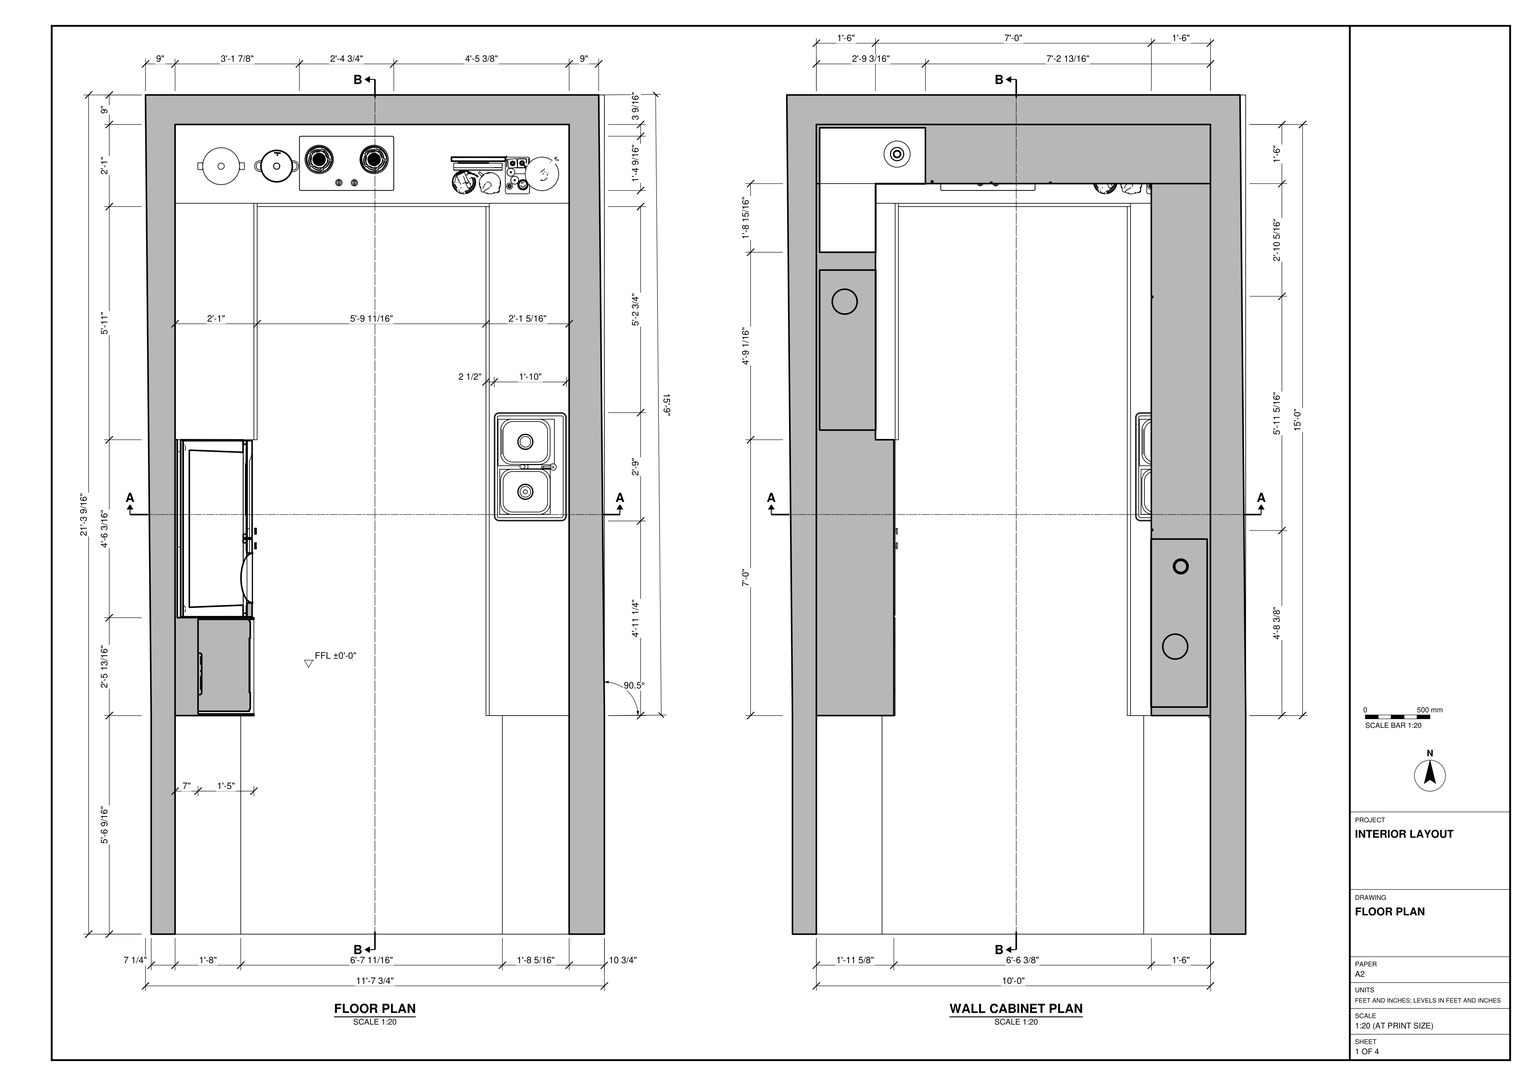
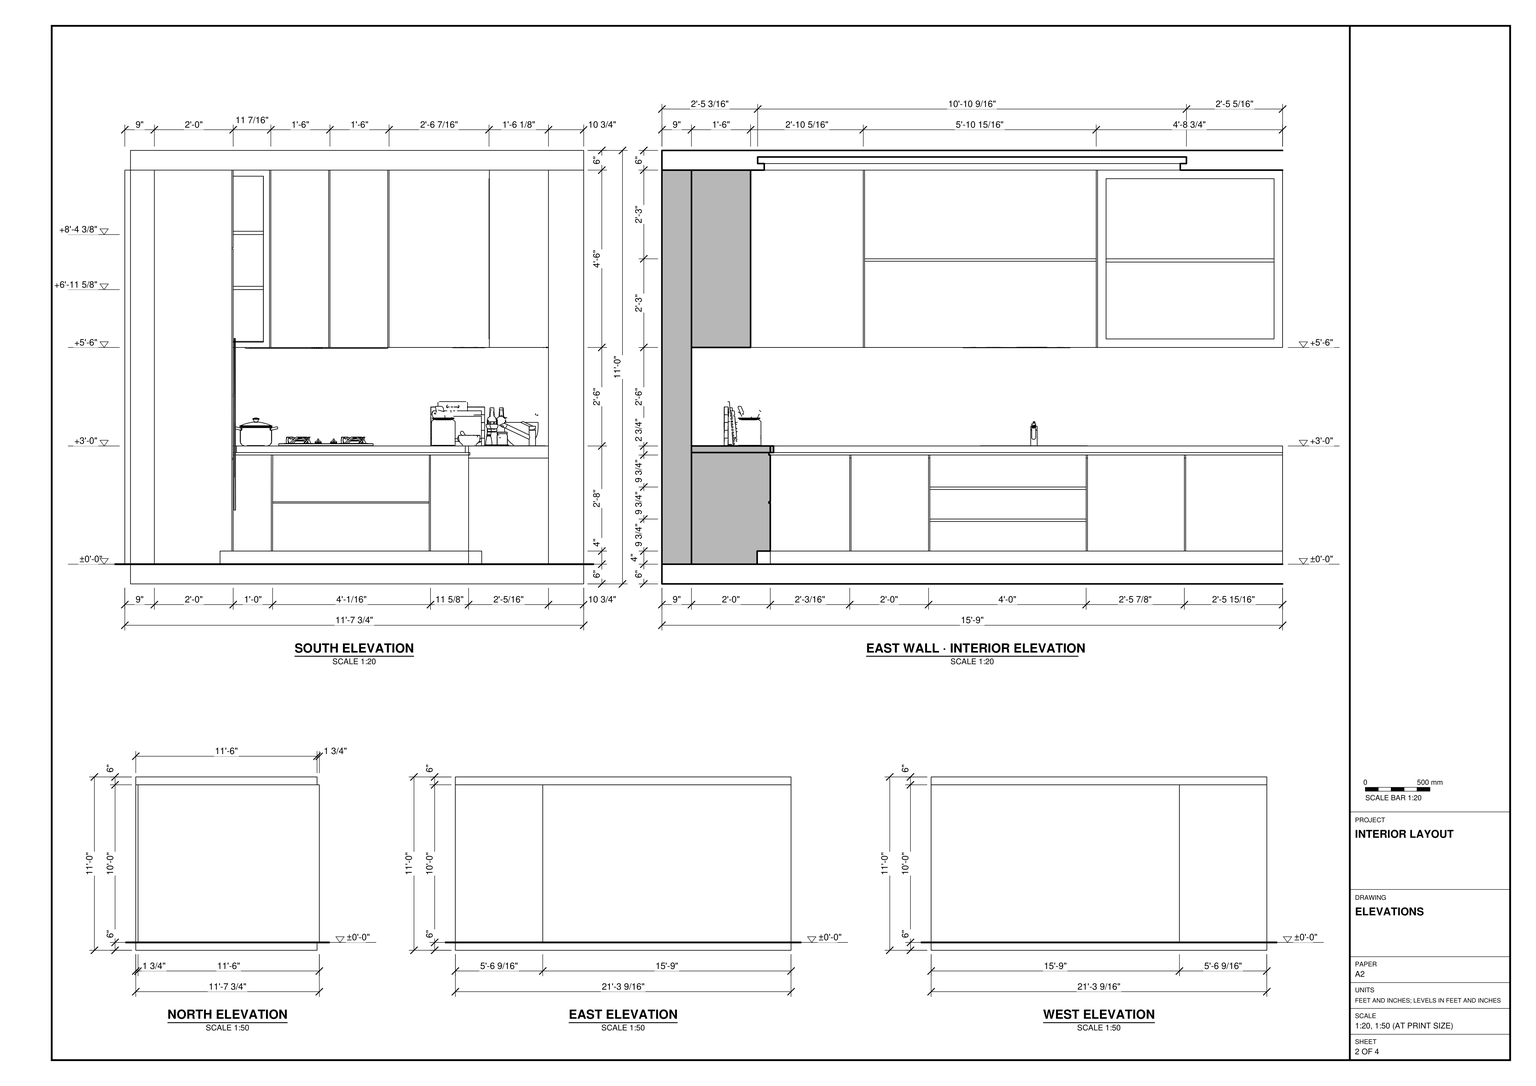
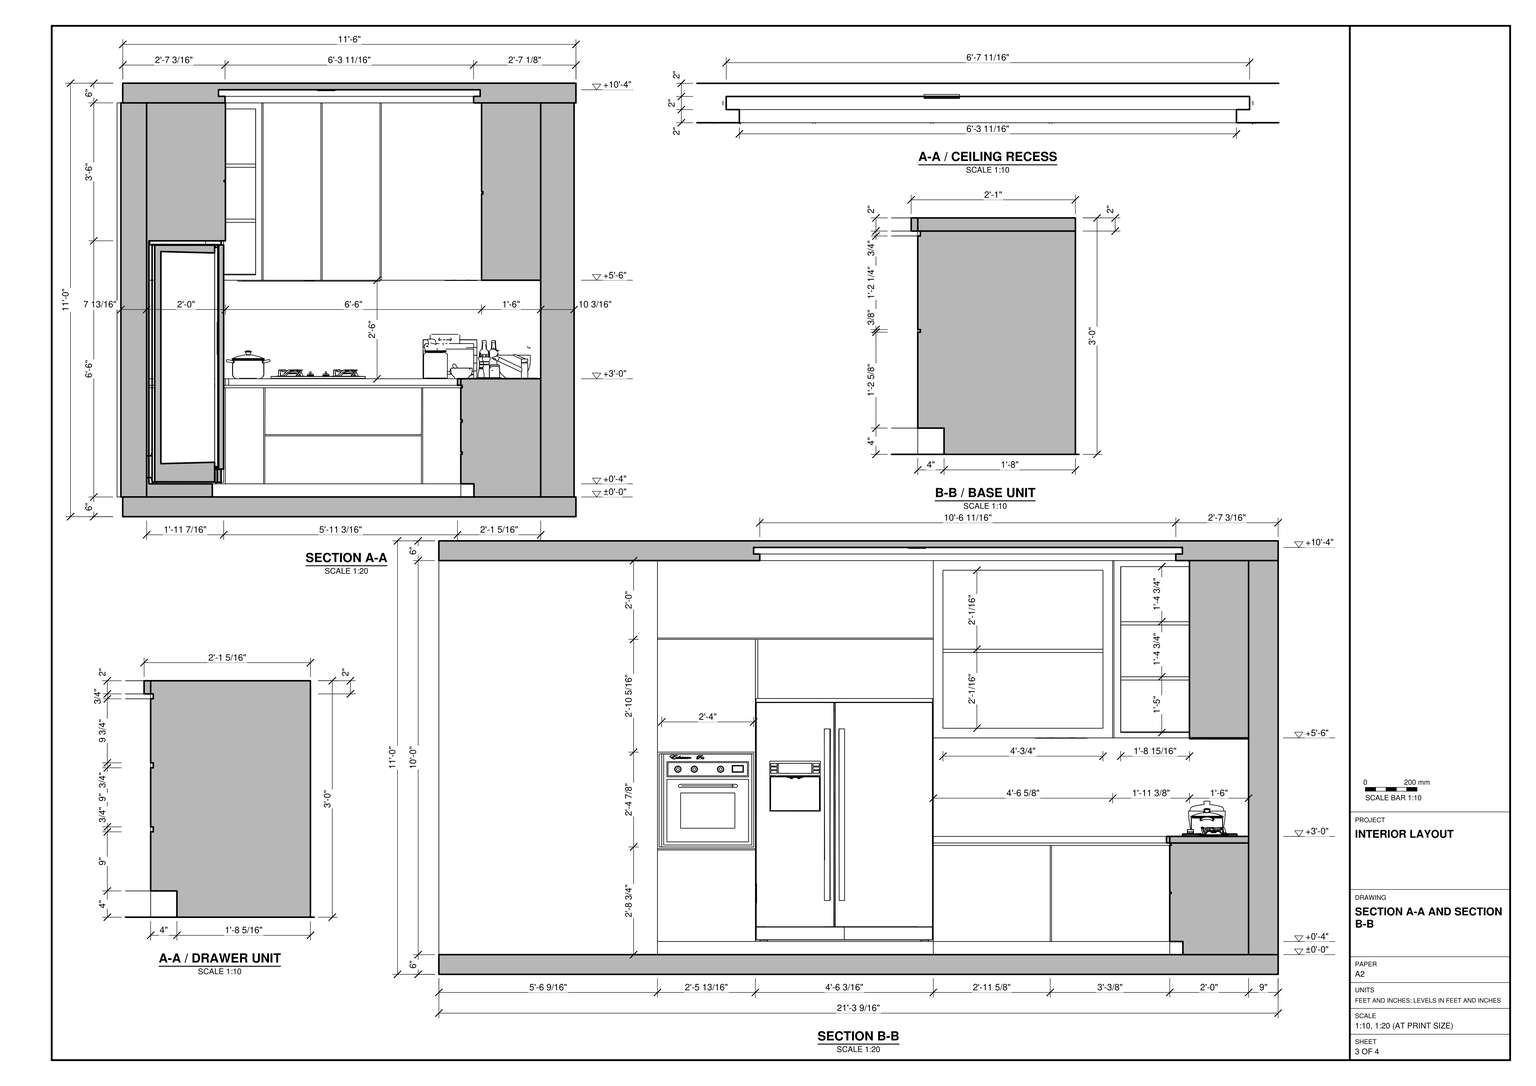
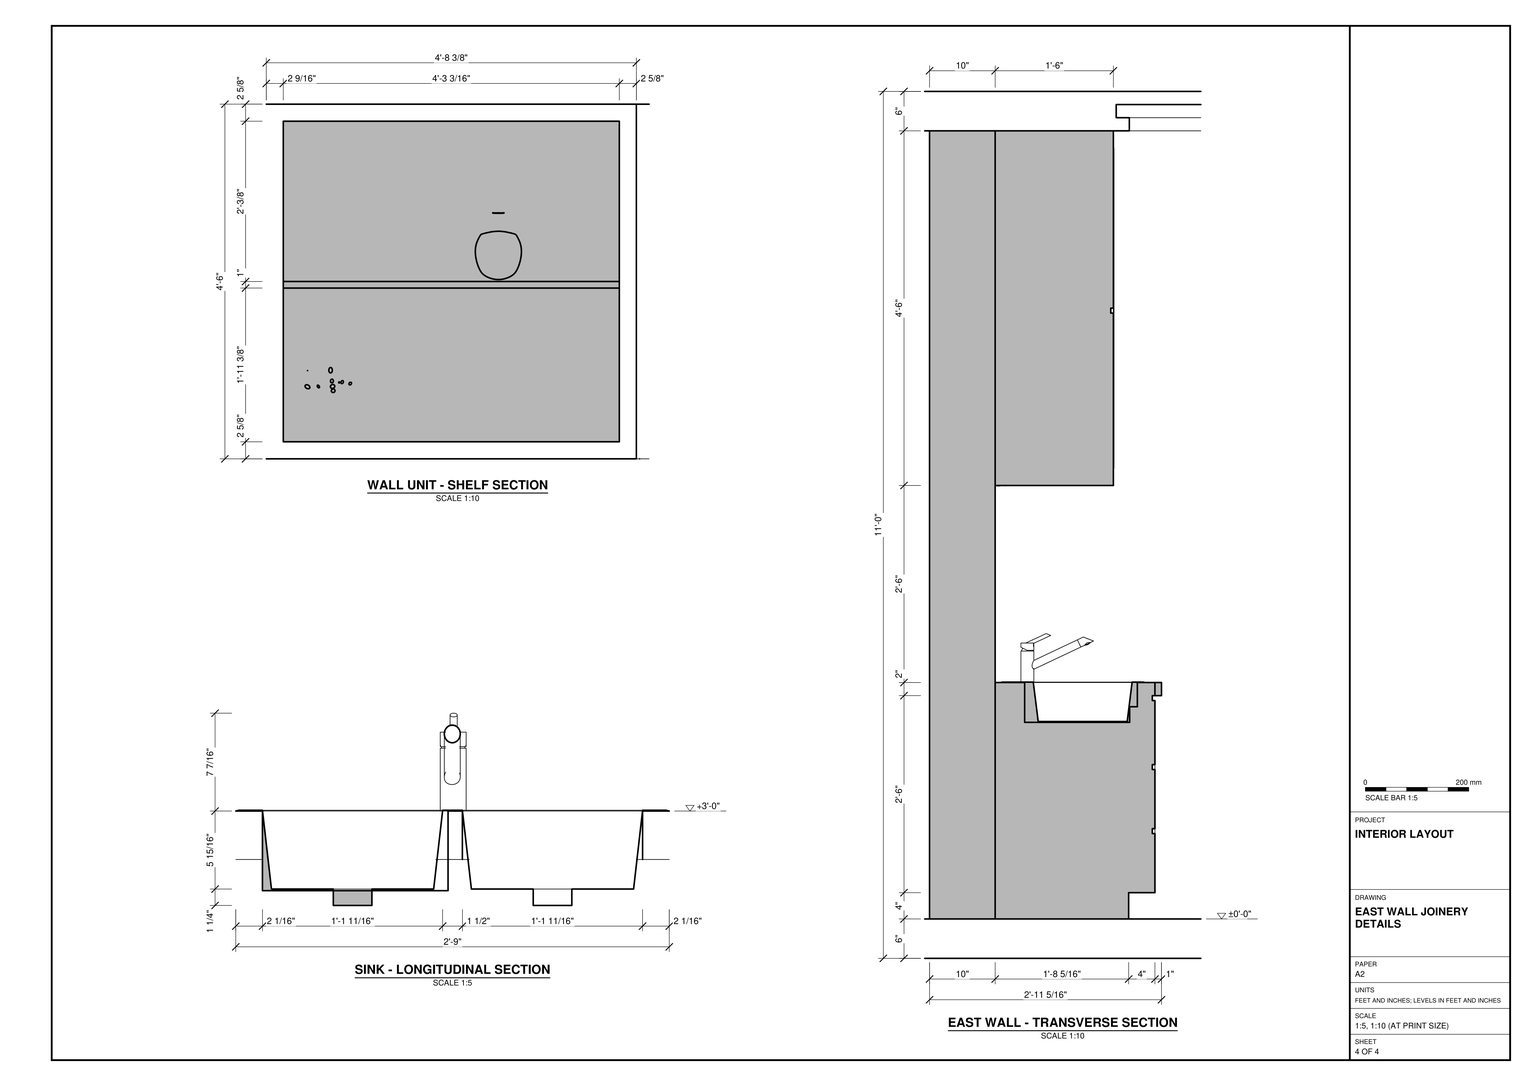
Build the kitchen interior in SketchUp using task_files/diagram_01.pdf. Work in feet and inches. The overall model is 11'-7 3/4" wide, 21'-3 9/16" long and 11'-0" high, with a single finished floor level at ±0'-0".

Model the floor slab, rear wall, side walls and ceiling slab. Follow the wall thicknesses and slight changes in alignment shown on the floor plan, leaving the front end open. Use the sections to form the stepped recess in the underside of the ceiling.

Fit the kitchen along the rear wall and both side walls, leaving the central aisle and the approach from the open end clear. Set the worktops at +3'-0". Place the cooktop on the rear run, the sink and tap on the right, and the tall oven and refrigerator bays on the left. Use the floor plan for the base units and the separate wall cabinet plan for the overhead units. Follow the elevations and sections for the drawer divisions, recessed plinths, cabinet fronts and open shelves. Appliances, cookware and other loose items may be any suitable library components.

Keep the walls, slabs and each joinery or furniture piece in separate groups or components, and use components for repeated parts. Save one SketchUp model as output_files/u_shaped_kitchen_with_cabinets_and_recessed_ceiling.skp.

# SketchUp Ruby script. Lengths in inches.
U = 1.inch
M = Sketchup.active_model
def pt(a) = Geom::Point3d.new(a.map { |v| v * U })
def face(e, loops, mat)
  f = e.add_face(loops[0].map { |a| pt(a) })
  loops[1..].each { |l| e.add_face(l.map { |a| pt(a) }).erase! }
  f.material = f.back_material = mat if mat
  f
end
# faces: each face lists its corners as indices into pts; further lists are holes
def faces(e, pts, list, mat = nil) = list.each { |f| face(e, (f[0].is_a?(Array) ? f : [f]).map { |l| l.map { |i| pts[i] } }, mat) }
# xy, xz, yz: faces in a plane at the given z, y or x. An outline is a flat list of corners, or four numbers for a rectangle; further outlines are holes
def ring(l) = l.size == 4 ? [[l[0], l[1]], [l[2], l[1]], [l[2], l[3]], [l[0], l[3]]] : l.each_slice(2).to_a
def flat(e, list, mat, &to3) = list.each { |f| face(e, (f[0].is_a?(Array) ? f : [f]).map { |l| ring(l).map { |u, v| to3.(u, v) } }, mat) }
def xy(e, z, list, mat = nil) = flat(e, list, mat) { |x, y| [x, y, z] }
def xz(e, y, list, mat = nil) = flat(e, list, mat) { |x, z| [x, y, z] }
def yz(e, x, list, mat = nil) = flat(e, list, mat) { |y, z| [x, y, z] }
def lines(e, pts, list) = list.each { |a, b| e.add_line(pt(pts[a]), pt(pts[b])) }
# prism: a flat outline (further loops are holes) pulled along v
def prism(e, loops, v, mat = nil)
  f = face(e, loops, mat); d = Geom::Vector3d.new(v.map { |x| x * U })
  f.pushpull(f.normal.samedirection?(d) ? d.length : -d.length)
end
def box(e, o, s, mat = nil) = prism(e, [[o, [o[0] + s[0], o[1], o[2]], [o[0] + s[0], o[1] + s[1], o[2]], [o[0], o[1] + s[1], o[2]]]], [0, 0, s[2]], mat)
def at(x, y, z, deg = 0) = Geom::Transformation.translation(pt([x, y, z])) * Geom::Transformation.rotation(ORIGIN, Z_AXIS, deg.degrees)
def axes(o, x, y, z) = Geom::Transformation.new([*x, 0, *y, 0, *z, 0, *pt(o).to_a, 1])
def part(name) = M.definitions.add(name)
# library, detail: a bought-in or finely detailed component or shape, given as its bounding box
def library(name, o, s) = part(name).tap { |d| box(d.entities, o, s) }
def detail(e, o, s) = box(e.add_group.entities, o, s)
def put(e, d, t, mat = nil) = e.add_instance(d, t).tap { |i| i.material = mat if mat }
def group(e, t, mat = nil) = e.add_group.tap { |g| g.transformation = t; g.material = mat if mat }.entities
root = M.entities
M.materials.add("Emissive").color = [239, 233, 180]
M.materials.add("Generic\#1").color = [204, 216, 199]
M.materials.add("Generic\#2").color = [83, 96, 74]
M.materials.add("Tiles Simple 02 100cm").color = [183, 183, 183]
M.materials.add("W147Z490B75_NILAYA MODERNISTA 32219 ROLL B75").color = [233, 234, 228]
M.materials.add("Whitewood Highgloss 300cm").color = [205, 205, 205]
M.materials.add("[Translucent Glass Gray]").color = [128, 128, 128]
M.materials["[Translucent Glass Gray]"].alpha = 0.5
M.materials.add("[Wood Veneer 02]").color = [186, 125, 89]
M.materials.add("[Wood Veneer 02]1").color = [188, 127, 90]
c1 = library("Untitled",[27.97,43.14,0],[33,22,16.3])
c2 = library("Rangemaaster flat hood",[-3.82,0.71,0],[43.23,19.01,40.35])
c3 = library("Lidded cooking pot",[0,0,0],[14.16,11.29,10.74])
c4 = part("Tlon Cubo 860 Ceiling 152 005")
xy(c4.entities,-3.04,[[-16.54,-16.54,-16.54,16.54,16.54,-16.54],[16.54,-16.54,-16.54,16.54,16.54,16.54]])
xy(c4.entities,0,[[-16.93,-16.93,16.93,-16.93,-16.93,16.93],[16.93,-16.93,16.93,16.93,-16.93,16.93]])
xz(c4.entities,-16.93,[[-16.93,-3.79,16.93,-3.79,-16.93,0],[16.93,-3.79,16.93,0,-16.93,0]])
xz(c4.entities,-16.3,[[-16.3,-3.66,-16.3,-3.24,16.3,-3.24],[-16.3,-3.66,16.3,-3.24,16.3,-3.66]])
xz(c4.entities,16.3,[[-16.3,-3.66,16.3,-3.24,-16.3,-3.24],[-16.3,-3.66,16.3,-3.66,16.3,-3.24]])
xz(c4.entities,16.93,[[-16.93,-3.79,-16.93,0,16.93,0],[-16.93,-3.79,16.93,0,16.93,-3.79]])
yz(c4.entities,-16.93,[[-16.93,-3.79,-16.93,0,16.93,0],[-16.93,-3.79,16.93,0,16.93,-3.79]])
yz(c4.entities,-16.3,[[-16.3,-3.66,16.3,-3.66,-16.3,-3.24],[16.3,-3.66,16.3,-3.24,-16.3,-3.24]])
yz(c4.entities,16.3,[[-16.3,-3.66,-16.3,-3.24,16.3,-3.66],[16.3,-3.66,-16.3,-3.24,16.3,-3.24]])
yz(c4.entities,16.93,[[-16.93,-3.79,16.93,-3.79,-16.93,0],[16.93,-3.79,16.93,0,-16.93,0]])
p = [[-16.93,-16.93,-3.79],[-16.93,16.93,-3.79],[-16.3,16.3,-3.66],[-16.3,-16.3,-3.66],[16.93,-16.93,-3.79],[16.3,-16.3,-3.66],
  [16.93,16.93,-3.79],[16.3,16.3,-3.66]]
faces(c4.entities,p,[[0,1,2],[2,3,0],[4,0,3],[3,5,4],[6,4,5],[5,7,6],[2,1,6],[6,7,2]])
c5 = library("Refrigerator 10-13",[-17.84,-12.49,0],[35.68,25.01,72.43])
c6 = library("kitchen utensils",[0,0,0],[25.84,8.08,11.16])
c7 = library("GasStove_Black",[0,0,0],[28.74,16.54,2.72])
c8 = library("现代小盆栽植物盆景多肉植物\#1",[493.55,-214.42,68.59],[116.32,134.38,44.63])
c9 = library("Kitchen oven",[-66.9,9.58,0],[22.04,24,22.83])
c10 = library("kitchen+utensil",[-39.88,-27.4,0],[79.77,28.4,32.96])
c11 = library("Kitchen Utensils - Pot",[14.77,-5.37,0.11],[13.29,9.84,8.54])
c12 = library("Gagri",[-4.64,1.37,-0.81],[22.18,22.19,29.95])
c13 = library("Group\#3",[-0.5,-0.5,0],[80.6875,131.5625,2])
c14 = part("Group\#34")
xy(c14.entities,0,[[0,0,0.1,48.73]])
xy(c14.entities,48.13,[[0,0,0.1,48.73]])
xz(c14.entities,0,[[0,0,0.1,9.0625],[0,9.0625,0.1,48.13]])
xz(c14.entities,48.73,[[0,0,0.1,48.13]])
yz(c14.entities,0,[[0,0,48.73,48.13]],"[Translucent Glass Gray]")
yz(c14.entities,0.1,[[0,0,48.73,48.13]],"[Translucent Glass Gray]")
c15 = library("Group\#35",[-0.5,-0.5,-0.1],[2,79,0.2])
c16 = library("Group\#36",[-0.5,-0.5,-0.1],[2,18,0.2])
c17 = library("Group\#82",[-0.5,-0.5,-0.1],[28.04,2,0.2])
c18 = library("Group\#83",[-0.5,-0.5,-0.1],[49.53,2,0.2])
c19 = library("Group\#84",[-0.5,-0.5,-0.1],[2,163,0.2])
xy(root,-6,[[1.73,0,139.73,255.5625]])
xy(root,0,[[1.73,0,9,0,9,246.5625,129,246.5625,129,0,139.73,0,139.73,66.5625,138,255.5625,1.73,255.5625],[9,0,29,66.5625],[108.67,0,129,66.5625],[1.73,66.5625,0,255.5625,1.73,255.5625],[9,66.5625,29,150.5625],
  [108.67,66.5625,129,222.5625],[139.73,66.5625,139.73,255.5625,138,255.5625],[9,150.5625,29,222.5625],[9,222.5625,29,222.5625,29,226.5625,108.67,226.5625,108.67,222.5625,129,222.5625,129,246.5625,9,246.5625]])
xy(root,0,[[29,0,108.67,226.5625]],"Whitewood Highgloss 300cm")
xy(root,4,[[9.6875,96.375,29,150.5625],[29,150.5625,29,222.5625,33,222.5625,33,186.5625,32.6,186.5625,32.6,186.16,33,186.16,33,150.5625],[29,222.5625,33,226.5625],[33,222.5625,33,226.5625,104.67,226.5625,104.67,222.5625,93.07,222.5625,93.07,222.96,92.67,222.96,92.67,222.5625,45,222.5625,45,222.96,44.6,222.96,44.6,222.5625],[104.67,222.5625,108.67,226.5625]])
xy(root,4,[[29,66.5625,33,96.375],[104.67,66.5625,104.67,96.07,105.07,96.07,105.07,96.47,104.67,96.47,104.67,125.98,105.07,125.98,105.07,126.375,104.67,126.375,104.67,173.98,105.07,173.98,105.07,174.375,104.67,174.375,104.67,197.98,105.07,197.98,105.07,198.375,104.67,198.375,104.67,222.5625,108.67,222.5625,108.67,66.5625]],"Generic\#1")
xy(root,13,[[104.67,126.375,105.07,173.98]])
xy(root,13.75,[[104.67,126.375,105.07,173.98]])
xy(root,18.6,[[45,222.5625,92.67,222.96]],"Generic\#2")
xy(root,19,[[45,222.5625,92.67,222.96]],"Generic\#2")
xy(root,22.75,[[104.67,126.375,105.07,173.98]])
xy(root,23.5,[[104.67,126.375,105.07,173.98]])
xy(root,29.9375,[[108.52,142.66,124.51,156.79]])
xy(root,31.875,[[32.6,66.5625,33,96.375]],"Generic\#2")
xy(root,32.27,[[32.6,66.5625,33,96.375]],"Generic\#2")
xy(root,32.3125,[[107.35,142.66,108.52,156.79],[104.67,222.5625,129,222.76]])
xy(root,32.78,[[16,67.07,33,95.87]],"Generic\#1")
xy(root,33.25,[[104.67,126.375,105.07,173.98],[32.6,150.5625,33,186.16],[32.6,222.5625,33,222.96],[33,222.5625,34,222.96],[45.06,222.5625,45.0625,222.96]])
xy(root,33.25,[[104.67,66.5625,105.07,96.07],[104.67,96.47,105.07,125.98],[104.67,174.375,105.07,197.98],[32.6,186.5625,33,222.5625],[104.67,198.375,105.07,222.96],
  [34,222.5625,44.6,222.96],[45.0625,222.5625,92.73,222.96],[93.07,222.5625,104.67,222.96]],"Generic\#2")
xy(root,34,[[9,150.5625,32.6,222.5625],[32.6,150.5625,33,222.5625],[9,222.5625,9,246.5625,129,246.5625,129,222.76,105.07,222.76,105.07,222.96,32.6,222.96,32.6,222.5625],[105.07,222.5625,129,222.76]])
xy(root,34,[[104.67,66.5625,105.07,222.5625],[32.6,222.5625,33,222.96],[33,222.5625,34,222.96],[34,222.5625,104.67,222.96],[104.67,222.5625,105.07,222.96]],"Generic\#2")
xy(root,34,[[103.67,66.5625,104.67,221.5625],[33,150.5625,34,222.5625],[34,221.5625,104.67,222.5625]],"Tiles Simple 02 100cm")
xy(root,36,[[103.67,66.5625,104.67,221.5625],[[104.67,66.5625,129,222.5625],[107.35,142.66,124.51,156.79],[107.85,127.85,123.25,141.57]],[9,150.5625,33,222.5625],[33,150.5625,34,222.5625],[34,221.5625,104.67,222.5625],
  [9,222.5625,129,246.5625]],"Tiles Simple 02 100cm")
xy(root,61.16,[[16,67.07,33,95.87]],"Generic\#1")
xy(root,66,[[111,66.5625,111,122.91,111.4,122.91,111.4,123.3125,111,123.3125,111,193.85,111.4,193.85,111.4,194.25,111,194.25,111,228.5625,128,228.5625,128,66.5625],[10,150.5625,27,228.5625],[10,228.5625,36.04,245.5625],[36.04,228.5625,36.04,246.5625,80.47,246.5625,80.47,245.5625,80.46,228.96,80.0625,228.96,80.0625,228.5625,62.46,228.5625,62.46,228.96,62.0625,228.96,62.0625,228.5625,44.46,228.5625,44.46,229.36,44.0625,229.36,44.0625,228.5625],[80.46,228.5625,80.46,228.96,80.47,245.5625,129,245.5625,129,228.5625]],"Generic\#1")
xy(root,67.85,[[10,207.65,27,228.5625],[10,228.5625,42.21,245.5625]],"[Wood Veneer 02]")
xy(root,68.59,[[110.9,69.16,111,120.32]])
xy(root,68.59,[[111,69.16,128,120.32]],"[Wood Veneer 02]")
xy(root,68.9375,[[10,153.5,27,202.23]],"[Wood Veneer 02]")
xy(root,78,[[9.6875,96.375,9.6875,150.5625,33,150.5625,33,97.125,32.6,97.125,32.6,96.375]])
xy(root,83.62,[[10,207.65,10.9,228.5625],[10,228.5625,10.9,245.5625],[10.9,244.66,42.21,245.5625]],"Emissive")
xy(root,83.62,[[10.9,207.65,27,228.5625],[10.9,228.5625,42.21,244.66]],"[Wood Veneer 02]")
xy(root,84.62,[[10,207.65,27,228.5625],[10,228.5625,42.21,245.5625]],"[Wood Veneer 02]")
xy(root,92,[[127.1,69.16,128,120.32],[10,153.5,10.9,202.23]],"Emissive")
xy(root,92,[[111,69.16,127.1,120.32],[10.9,153.5,27,202.23]],"[Wood Veneer 02]")
xy(root,92.25,[[111,123.3125,111.4,193.85]],"Generic\#2")
xy(root,93,[[111,123.3125,111.4,193.85]],"Generic\#2")
xy(root,93,[[111,69.16,128,120.32],[10,153.5,27,202.23]],"[Wood Veneer 02]")
xy(root,96,[[32.6,66.5625,33,96.375],[32.6,97.125,33,150.5625]],"Generic\#2")
xy(root,96.4,[[32.6,66.5625,33,96.375],[32.6,96.375,33,150.5625]],"Generic\#2")
xy(root,100.38,[[10,207.65,10.9,228.5625],[10,228.5625,10.9,245.5625],[10.9,244.66,42.21,245.5625]],"Emissive")
xy(root,100.38,[[10.9,207.65,27,228.5625],[10.9,228.5625,42.21,244.66]],"[Wood Veneer 02]")
xy(root,101.38,[[10,207.65,27,228.5625],[10,228.5625,42.21,245.5625]],"[Wood Veneer 02]")
xy(root,117.0625,[[10,153.5,10.9,202.23]],"Emissive")
xy(root,117.0625,[[10.9,153.5,27,202.23]],"[Wood Veneer 02]")
xy(root,117.41,[[110.9,69.16,111,120.32]])
xy(root,117.41,[[127.1,69.16,128,120.32]],"Emissive")
xy(root,117.41,[[111,69.16,127.1,120.32]],"[Wood Veneer 02]")
xy(root,118.15,[[10,207.65,10.9,228.5625],[10,228.5625,10.9,245.5625],[10.9,244.66,42.21,245.5625]],"Emissive")
xy(root,118.15,[[10.9,207.65,27,228.5625],[10.9,228.5625,42.21,244.66]],"[Wood Veneer 02]")
xy(root,120,[[1.73,0,1.73,255.5625,138,255.5625,139.73,66.5625,139.73,0,129,0,129,246.5625,9,246.5625,9,0],[9,0,32.6,66.5625],[32.6,0,33,66.5625],[111,0,129,66.5625],[1.73,66.5625,1.73,255.5625,0,255.5625],
  [9,66.5625,33,66.5625,33,97.72,32.89,97.72,32.89,150.5625,9,150.5625],[111,66.5625,111,122.91,111.4,122.91,111.4,123.3125,111,123.3125,111,193.85,111.4,193.85,111.4,194.25,111,194.25,111,228.5625,129,228.5625,129,66.5625],[139.73,66.5625,138,255.5625,139.73,255.5625],[32.89,97.72,33,150.5625],[9,150.5625,27,228.5625],
  [9,228.5625,44.0625,228.5625,44.0625,229.36,44.46,229.36,44.46,228.5625,62.0625,228.5625,62.0625,228.96,62.46,228.96,62.46,228.5625,80.0625,228.5625,80.0625,228.96,80.46,228.96,80.46,228.5625,129,228.5625,129,246.5625,9,246.5625]])
xy(root,120,[[[33,0,33,66.5625,9,66.5625,9,246.5625,129,246.5625,129,228.5625,111,228.5625,111,194.25,111.4,194.25,111.4,193.85,111,193.85,111,123.3125,111.4,123.3125,111.4,122.91,111,122.91,111,0],[32.89,97.72,108.57,224.41]]],"W147Z490B75_NILAYA MODERNISTA 32219 ROLL B75")
xy(root,122,[[30.89,95.84,32.89,224.41],[32.89,95.84,110.57,97.72],[108.57,97.72,110.57,224.41],[30.89,224.41,110.57,226.41]])
xy(root,124,[[30.89,95.84,110.57,226.41]],"W147Z490B75_NILAYA MODERNISTA 32219 ROLL B75")
xy(root,126,[[1.73,0,139.73,255.5625]])
xz(root,0,[[1.73,-6,139.73,0],[1.73,0,9,120],[129,0,139.73,120],[1.73,120,139.73,126]])
xz(root,66.5625,[[32.6,96.4,33,120]])
xz(root,66.5625,[[9,0,29,0,29,4,32.6,4,32.6,120,9,120],[108.67,0,129,0,129,32.3125,104.67,32.3125,104.67,4,108.67,4],[111,66,129,120]],"Generic\#1")
xz(root,66.5625,[[32.6,4,33,31.875],[32.6,32.27,33,96]],"Generic\#2")
xz(root,66.5625,[[104.67,32.3125,129,32.3125,129,36,104.67,36,104.67,34,105.07,34,105.07,33.25,104.67,33.25],[103.67,34,104.67,36]],"Tiles Simple 02 100cm")
xz(root,67.07,[[16,32.78,33,61.16]],"Generic\#1")
xz(root,69.16,[[110.9,68.59,111,117.41],[111,92,128,93]])
xz(root,69.16,[[111,68.59,128,92],[111,93,128,117.41]],"[Wood Veneer 02]")
xz(root,95.87,[[16,32.78,33,61.16]],"Generic\#1")
xz(root,96.07,[[104.67,4,105.07,32.3125],[104.67,32.3125,105.07,33.25]],"Generic\#2")
xz(root,96.375,[[9.6875,4,9.6875,78,33,78,33,32.27,32.6,32.27,32.6,31.875,33,31.875,33,4]])
xz(root,96.375,[[32.6,78,33,96]],"Generic\#2")
xz(root,96.47,[[104.67,4,105.07,32.3125],[104.67,32.3125,105.07,33.25]],"Generic\#2")
xz(root,97.125,[[32.6,78,33,96]],"Generic\#2")
xz(root,97.72,[[32.89,120,108.57,122]])
xz(root,120.32,[[110.9,68.59,111,117.41],[111,92,128,93]])
xz(root,120.32,[[111,68.59,128,92],[111,93,128,117.41]],"[Wood Veneer 02]")
xz(root,122.91,[[111,66,111.4,120]],"Generic\#2")
xz(root,123.3125,[[111,66,111.4,92.25],[111,93,111.4,120]],"Generic\#2")
xz(root,125.98,[[104.67,4,105.07,32.3125],[104.67,32.3125,105.07,33.25]])
xz(root,126.375,[[104.67,4,105.07,13],[104.67,13.75,105.07,22.75],[104.67,23.5,105.07,32.3125],[104.67,32.3125,105.07,33.25]])
xz(root,127.85,[[107.85,32.3125,123.25,36]])
xz(root,141.57,[[107.85,32.3125,123.25,36]])
xz(root,142.66,[[108.52,29.9375,124.51,32.3125],[107.35,32.3125,124.51,36]])
xz(root,150.5625,[[9,0,9,34,9.6875,34,9.6875,4,29,4,29,0],[9.6875,4,33,33.25],[9.6875,33.25,32.6,34],[9,34,9.6875,36],[9.6875,34,33,36],
  [33,34,34,36],[9,36,9.6875,66],[9.6875,66,27,78],[27,78,29,120],[29,78,29,120,33,120,33,96.4,32.6,96.4,32.6,96,33,96,33,78]])
xz(root,153.5,[[10,68.9375,27,78],[10,78,27,92],[10,93,27,117.0625]],"[Wood Veneer 02]")
xz(root,156.79,[[108.52,29.9375,124.51,32.3125],[107.35,32.3125,124.51,36]])
xz(root,173.98,[[104.67,4,105.07,13],[104.67,13.75,105.07,22.75],[104.67,23.5,105.07,32.3125],[104.67,32.3125,105.07,33.25]])
xz(root,174.375,[[104.67,4,105.07,32.3125],[104.67,32.3125,105.07,33.25]])
xz(root,186.16,[[32.6,4,33,33.25]],"Generic\#2")
xz(root,186.5625,[[32.6,4,33,33.25]],"Generic\#2")
xz(root,193.85,[[111,66,111.4,92.25],[111,93,111.4,120]],"Generic\#2")
xz(root,194.25,[[111,66,111.4,120]],"Generic\#2")
xz(root,197.98,[[104.67,4,105.07,32.3125],[104.67,32.3125,105.07,33.25]],"Generic\#2")
xz(root,198.375,[[104.67,4,105.07,32.3125],[104.67,32.3125,105.07,33.25]],"Generic\#2")
xz(root,202.23,[[10,68.9375,27,92],[10,93,27,117.0625]],"[Wood Veneer 02]")
xz(root,207.65,[[10,67.85,27,83.62],[10,84.62,27,100.38],[10,101.38,27,118.15]])
xz(root,221.5625,[[103.67,34,104.67,36]])
xz(root,221.5625,[[34,34,103.67,36]],"Tiles Simple 02 100cm")
xz(root,222.5625,[[9,0,9,34,32.6,34,32.6,33.25,33,33.25,33,4,29,4,29,0],[108.67,0,129,0,129,32.3125,104.67,32.3125,104.67,4,108.67,4],[9,34,33,36],[33,34,34,36],[34,34,104.67,36],
  [104.67,34,129,36]])
xz(root,222.5625,[[33,4,44.6,33.25],[45,4,92.67,18.6],[93.07,4,104.67,33.25],[45,19,92.67,19,92.73,33.25,45.06,33.25]],"Generic\#1")
xz(root,222.96,[[44.6,4,45,4,45,19,45.06,33.25,44.6,33.25],[92.67,4,93.07,4,93.07,33.25,92.73,33.25,92.67,19],[45,18.6,92.67,19],[32.6,33.25,104.67,34],[104.67,33.25,105.07,34]],"Generic\#2")
xz(root,224.41,[[32.89,120,108.57,122]],"W147Z490B75_NILAYA MODERNISTA 32219 ROLL B75")
xz(root,226.5625,[[29,0,104.67,4],[104.67,0,108.67,4]],"Generic\#1")
xz(root,228.5625,[[9,66,9,120,27,120,27,118.15,10,118.15,10,101.38,27,101.38,27,100.38,10,100.38,10,84.62,27,84.62,27,83.62,10,83.62,10,67.85,27,67.85,27,66],[111,66,129,120]])
xz(root,228.5625,[[44.46,66,62.0625,120],[62.46,66,80.0625,120],[80.46,66,111,120]],"Generic\#1")
xz(root,228.5625,[[27,66,44.0625,66,44.0625,120,27,120,27,118.15,42.21,118.15,42.21,67.85,27,67.85]],"Generic\#2")
xz(root,228.5625,[[27,83.62,42.21,84.62],[27,100.38,42.21,101.38]],"[Wood Veneer 02]")
xz(root,228.96,[[62.0625,66,62.46,120],[80.0625,66,80.46,120]],"Generic\#2")
xz(root,229.36,[[44.0625,66,44.46,120]],"Generic\#2")
xz(root,245.5625,[[10,67.85,42.21,83.62],[10,84.62,42.21,100.38],[10,101.38,42.21,118.15]],"[Wood Veneer 02]")
xz(root,246.5625,[[9,0,129,34],[9,34,129,36],[9,66,129,120]])
xz(root,246.5625,[[9,36,129,66]],"Generic\#2")
xz(root,255.5625,[[1.73,-6,139.73,0],[0,0,138,120],[1.73,120,139.73,126]])
yz(root,1.73,[[0,-6,255.5625,0],[0,0,66.5625,120],[0,120,255.5625,126]])
yz(root,9,[[0,0,66.5625,120],[66.5625,0,150.5625,120],[150.5625,0,222.5625,34],[222.5625,0,246.5625,34],[150.5625,34,222.5625,36],
  [222.5625,34,246.5625,36],[150.5625,66,228.5625,120],[228.5625,66,246.5625,120]])
yz(root,9,[[150.5625,36,246.5625,66]],"Generic\#2")
yz(root,9.6875,[[96.375,4,150.5625,78]])
yz(root,10,[[207.65,67.85,228.5625,83.62],[228.5625,67.85,245.5625,83.62],[153.5,68.9375,202.23,92],[207.65,84.62,228.5625,100.38],[228.5625,84.62,245.5625,100.38],
  [153.5,93,202.23,117.0625],[207.65,101.38,228.5625,118.15],[228.5625,101.38,245.5625,118.15]],"[Wood Veneer 02]")
yz(root,16,[[67.07,32.78,95.87,61.16]],"Generic\#1")
yz(root,27,[[205.16,66,205.5625,120]])
yz(root,27,[[[150.5625,66,205.16,120],[153.5,68.9375,202.23,117.0625]],[205.5625,66,228.5625,66,228.5625,67.85,207.65,67.85,207.65,118.15,228.5625,118.15,228.5625,120,205.5625,120]],"Generic\#2")
yz(root,27,[[207.65,83.62,228.5625,84.62],[153.5,92,202.23,93],[207.65,100.38,228.5625,101.38]],"[Wood Veneer 02]")
yz(root,29,[[66.5625,0,150.5625,4],[150.5625,0,222.5625,4],[222.5625,0,226.5625,4]],"Generic\#1")
yz(root,32.6,[[186.16,4,186.5625,33.25],[66.5625,31.875,96.375,32.27],[150.5625,33.25,222.5625,34],[222.5625,33.25,222.96,34],[96.375,78,97.125,96],
  [66.5625,96,150.5625,96.4]],"Generic\#2")
yz(root,32.89,[[97.72,120,224.41,122]],"W147Z490B75_NILAYA MODERNISTA 32219 ROLL B75")
yz(root,33,[[150.5625,34,222.5625,36]])
yz(root,33,[[66.5625,4,96.375,31.875],[150.5625,4,186.16,33.25],[186.5625,4,222.5625,33.25],[[66.5625,32.27,96.375,61.67],[67.07,32.78,95.87,61.16]],[66.5625,61.67,96.375,96],
  [97.125,78,150.5625,96],[66.5625,96.4,150.5625,120]],"Generic\#1")
yz(root,34,[[221.5625,34,222.5625,36]])
yz(root,34,[[150.5625,34,221.5625,36]],"Tiles Simple 02 100cm")
yz(root,42.21,[[228.5625,100.38,245.5625,101.38]])
yz(root,42.21,[[228.5625,67.85,245.5625,83.62],[228.5625,84.62,245.5625,100.38],[228.5625,101.38,245.5625,118.15]],"[Wood Veneer 02]1")
yz(root,44.0625,[[228.5625,66,229.36,120]],"Generic\#2")
yz(root,44.46,[[228.5625,66,229.36,120]],"Generic\#2")
yz(root,44.6,[[222.5625,4,222.96,19],[222.5625,19,222.96,33.25]],"Generic\#2")
yz(root,45,[[222.5625,4,222.96,18.6]])
yz(root,62.0625,[[228.5625,66,228.96,120]],"Generic\#2")
yz(root,62.46,[[228.5625,66,228.96,120]],"Generic\#2")
yz(root,80.0625,[[228.5625,66,228.96,120]],"Generic\#2")
yz(root,80.46,[[228.5625,66,228.96,120]],"Generic\#2")
yz(root,92.67,[[222.5625,4,222.96,18.6]],"Generic\#2")
yz(root,93.07,[[222.5625,4,222.96,19],[222.5625,19,222.96,33.25]],"Generic\#2")
yz(root,103.67,[[66.5625,34,221.5625,36]],"Tiles Simple 02 100cm")
yz(root,104.67,[[222.5625,32.3125,222.76,33.25],[66.5625,34,221.5625,36],[221.5625,34,222.5625,36]])
yz(root,104.67,[[66.5625,4,96.07,33.25],[96.47,4,125.98,33.25],[126.375,4,173.98,13],[174.375,4,197.98,33.25],[198.375,4,222.5625,33.25],
  [126.375,13.75,173.98,22.75],[126.375,23.5,173.98,33.25]],"Generic\#1")
yz(root,105.07,[[125.98,4,126.375,32.3125],[173.98,4,174.375,32.3125],[126.375,13,173.98,13.75],[126.375,22.75,173.98,23.5],[125.98,32.3125,126.375,33.25],
  [173.98,32.3125,174.375,33.25]])
yz(root,105.07,[[96.07,4,96.47,32.3125],[197.98,4,198.375,32.3125],[96.07,32.3125,96.47,33.25],[197.98,32.3125,198.375,33.25],[66.5625,33.25,222.96,34]],"Generic\#2")
yz(root,107.35,[[142.66,32.3125,156.79,36]])
yz(root,107.85,[[127.85,32.3125,141.57,36]])
yz(root,108.52,[[142.66,29.9375,156.79,32.3125]])
yz(root,108.57,[[97.72,120,224.41,122]],"W147Z490B75_NILAYA MODERNISTA 32219 ROLL B75")
yz(root,108.67,[[222.5625,0,226.5625,4]])
yz(root,108.67,[[66.5625,0,222.5625,4]],"Generic\#1")
yz(root,110.9,[[69.16,68.59,120.32,117.41]],"[Translucent Glass Gray]")
yz(root,111,[[123.3125,66,193.85,92.25],[194.25,66,228.5625,120],[123.3125,93,193.85,120]],"Generic\#1")
yz(root,111,[[[66.5625,66,122.91,120],[69.16,68.59,120.32,117.41]]],"Generic\#2")
yz(root,111,[[69.16,68.59,120.32,92],[69.16,93,120.32,117.41]],"[Translucent Glass Gray]")
yz(root,111,[[69.16,92,120.32,93]],"[Wood Veneer 02]")
yz(root,111.4,[[122.91,66,123.3125,120],[193.85,66,194.25,120],[123.3125,92.25,193.85,93]],"Generic\#2")
yz(root,123.25,[[127.85,32.3125,141.57,36]])
yz(root,124.51,[[142.66,29.9375,156.79,32.3125],[142.66,32.3125,156.79,36]])
yz(root,128,[[69.16,92,120.32,93]])
yz(root,128,[[69.16,68.59,120.32,92],[69.16,93,120.32,117.41]],"[Wood Veneer 02]")
yz(root,129,[[0,0,66.5625,32.3125],[66.5625,0,222.5625,32.3125],[222.5625,0,222.5625,32.3125,222.76,32.3125,222.76,34,246.5625,34,246.5625,0],[0,32.3125,66.5625,36],[66.5625,32.3125,66.5625,36,222.5625,36,222.5625,34,222.76,34,222.76,32.3125],
  [222.5625,34,246.5625,36],[0,66,66.5625,120],[66.5625,66,228.5625,120],[228.5625,66,246.5625,120]])
yz(root,129,[[0,36,246.5625,66]],"Generic\#2")
yz(root,139.73,[[0,-6,255.5625,0],[0,0,66.5625,120],[0,120,255.5625,126]])
p = [[0,255.5625,0],[1.73,66.5625,0],[1.73,66.5625,120],[0,255.5625,120],[139.73,66.5625,0],[138,255.5625,0],
  [138,255.5625,120],[139.73,66.5625,120],[45,222.5625,19],[45.06,222.5625,33.25],[45.06,222.96,33.25],[45,222.96,19],
  [92.73,222.5625,33.25],[92.67,222.5625,19],[92.67,222.96,19],[92.73,222.96,33.25]]
faces(root,p,[[0,1,2,3],[4,5,6,7]])
faces(root,p,[[8,9,10,11],[12,13,14,15]],"Generic\#2")
put(root,c1,at(171.3125,97.85,27.5625,90))
put(root,c2,axes([40.65,227.89,65.7],[1,0,0],[0,0.94658,0],[0,0,0.11]))
put(root,c3,at(15.93,228.22,36))
put(root,c4,axes([63.71,145.5625,124.3],[0.16,0,0],[0,0.16,0],[0,0,0.16]))
put(root,c5,axes([21.375,123.47,4],[0,1.51901,0],[-0.9886,0,0],[0,0,1.02161]))
put(root,c6,at(15.09,233.01,67.85))
put(root,c7,at(46.87,226.46,36))
put(root,c8,at(-482.03,320.27,0))
put(root,c9,axes([39.78,152.84,32.78],[0,1.27,0],[-0.70823,0,0],[0,0,1.26502]))
put(root,c10,axes([109.52,236.61,36],[0.41,0,0],[0,0.41,0],[0,0,0.41]))
put(root,c11,at(18.51,234.34,35.89))
put(root,c12,axes([31.26,233.05,84.91],[0.36,0,0],[0,0.36,0],[0,0,0.36]))
put(root,c12,axes([15.3125,188.12,93.29],[0.36,0,0],[0,0.36,0],[0,0,0.36]))
put(root,c12,axes([115.95,83.09,93.29],[0.36,0,0],[0,0.36,0],[0,0,0.36]))
put(root,c13,at(30.89,95.84,122))
put(root,c14,at(27,153.5,68.9375))
put(root,c14,axes([27,207.61,67.62],[1,0,0],[0,0.43,0],[0,0,1.05]))
put(root,c14,axes([42.1875,228.46,67.62],[0,1,0],[-0.3096,0,0],[0,0,1.05]))
put(root,c15,at(9,150.5625,66))
put(root,c16,at(9,228.5625,66))
put(root,c17,at(9,245.5625,66))
put(root,c18,at(80.47,245.5625,66))
put(root,c19,at(128,66.5625,66))
